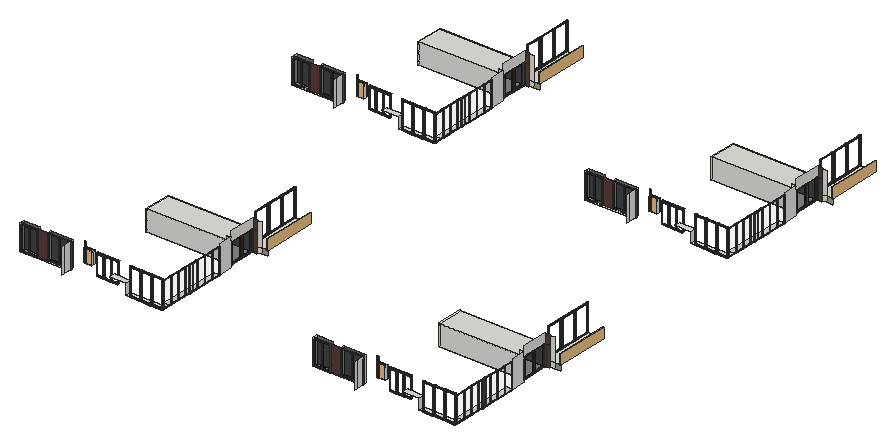
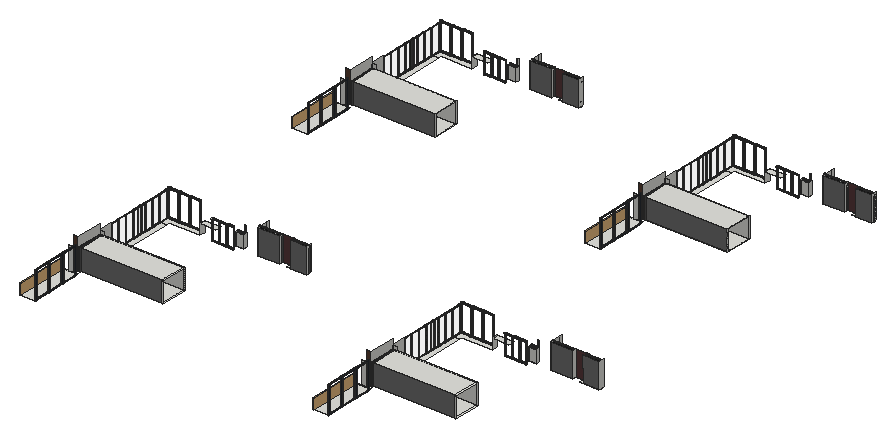
# SketchUp Ruby script. Lengths in inches.
U = 1.inch
M = Sketchup.active_model
def pt(a) = Geom::Point3d.new(a.map { |v| v * U })
def face(e, loops, mat)
  f = e.add_face(loops[0].map { |a| pt(a) })
  loops[1..].each { |l| e.add_face(l.map { |a| pt(a) }).erase! }
  f.material = f.back_material = mat if mat
  f
end
# faces: each face lists its corners as indices into pts; further lists are holes
def faces(e, pts, list, mat = nil) = list.each { |f| face(e, (f[0].is_a?(Array) ? f : [f]).map { |l| l.map { |i| pts[i] } }, mat) }
# xy, xz, yz: faces in a plane at the given z, y or x. An outline is a flat list of corners, or four numbers for a rectangle; further outlines are holes
def ring(l) = l.size == 4 ? [[l[0], l[1]], [l[2], l[1]], [l[2], l[3]], [l[0], l[3]]] : l.each_slice(2).to_a
def flat(e, list, mat, &to3) = list.each { |f| face(e, (f[0].is_a?(Array) ? f : [f]).map { |l| ring(l).map { |u, v| to3.(u, v) } }, mat) }
def xy(e, z, list, mat = nil) = flat(e, list, mat) { |x, y| [x, y, z] }
def xz(e, y, list, mat = nil) = flat(e, list, mat) { |x, z| [x, y, z] }
def yz(e, x, list, mat = nil) = flat(e, list, mat) { |y, z| [x, y, z] }
def lines(e, pts, list) = list.each { |a, b| e.add_line(pt(pts[a]), pt(pts[b])) }
# prism: a flat outline (further loops are holes) pulled along v
def prism(e, loops, v, mat = nil)
  f = face(e, loops, mat); d = Geom::Vector3d.new(v.map { |x| x * U })
  f.pushpull(f.normal.samedirection?(d) ? d.length : -d.length)
end
def box(e, o, s, mat = nil) = prism(e, [[o, [o[0] + s[0], o[1], o[2]], [o[0] + s[0], o[1] + s[1], o[2]], [o[0], o[1] + s[1], o[2]]]], [0, 0, s[2]], mat)
def at(x, y, z, deg = 0) = Geom::Transformation.translation(pt([x, y, z])) * Geom::Transformation.rotation(ORIGIN, Z_AXIS, deg.degrees)
def axes(o, x, y, z) = Geom::Transformation.new([*x, 0, *y, 0, *z, 0, *pt(o).to_a, 1])
def part(name) = M.definitions.add(name)
# library, detail: a bought-in or finely detailed component or shape, given as its bounding box
def library(name, o, s) = part(name).tap { |d| box(d.entities, o, s) }
def detail(e, o, s) = box(e.add_group.entities, o, s)
def put(e, d, t, mat = nil) = e.add_instance(d, t).tap { |i| i.material = mat if mat }
def group(e, t, mat = nil) = e.add_group.tap { |g| g.transformation = t; g.material = mat if mat }.entities
root = M.entities
M.materials.add("Glass_Tinted_Gray").color = [0, 0, 0]
M.materials["Glass_Tinted_Gray"].alpha = 0.125
M.materials.add("Glazing").color = [128, 128, 128]
M.materials["Glazing"].alpha = 0.05
M.materials.add("Powdercoating").color = [41, 44, 40]
M.materials.add("Wine2").color = [0, 0, 0]
M.materials["Wine2"].alpha = 0
M.materials.add("[0130_Gainsboro]").color = [39, 45, 50]
M.materials.add("[0135_DarkGray]").color = [81, 81, 81]
M.materials.add("[Color M05]").color = [114, 114, 114]
M.materials.add("[Color M06]").color = [86, 86, 86]
M.materials.add("[Concrete Tile]").color = [165, 155, 133]
M.materials.add("[Granite Brown]").color = [89, 59, 61]
M.materials.add("[Granite Brown]1").color = [89, 63, 50]
M.materials.add("[Mirror 02]").color = [229, 229, 229]
M.materials.add("[Terrazzo Light Blue]").color = [196, 214, 227]
c1 = part("Group\#15")
xy(c1.entities,0,[[0,-55.94,0.71,45.94]])
xy(c1.entities,0.2,[[0,-55.94,0.47,45.94],[0.47,45.94,0.71,46.42]])
xy(c1.entities,2.36,[[0.47,-55.94,0.71,46.42]])
xz(c1.entities,-55.94,[[0,0,0.71,0,0.71,2.36,0.47,2.36,0.47,0.2,0,0.2]])
xz(c1.entities,45.94,[[0,0,0.71,0.2]])
xz(c1.entities,46.42,[[0.47,0.2,0.71,2.36]])
yz(c1.entities,0,[[-55.94,0,45.94,0.2]])
yz(c1.entities,0.47,[[-55.94,0.2,46.42,2.36]])
yz(c1.entities,0.71,[[-55.94,0,45.94,0,45.94,0.2,46.42,0.2,46.42,2.36,-55.94,2.36]])
c2 = part("Group\#7")
xy(c2.entities,0,[[0,-59.09,0.71,45.94]])
xy(c2.entities,0.2,[[0,-59.09,0.47,45.94],[0.47,45.94,0.71,46.42]])
xy(c2.entities,2.36,[[0.47,-59.09,0.71,46.42]])
xz(c2.entities,-59.09,[[0,0,0.71,0,0.71,2.36,0.47,2.36,0.47,0.2,0,0.2]])
xz(c2.entities,45.94,[[0,0,0.71,0.2]])
xz(c2.entities,46.42,[[0.47,0.2,0.71,2.36]])
yz(c2.entities,0,[[-59.09,0,45.94,0.2]])
yz(c2.entities,0.47,[[-59.09,0.2,46.42,2.36]])
yz(c2.entities,0.71,[[-59.09,0,45.94,0,45.94,0.2,46.42,0.2,46.42,2.36,-59.09,2.36]])
c3 = part("Group\#16")
prism(c3.entities,[[[0.47,-56.18,0.2],[0,-56.18,0.2],[0,-56.18,0],[0.71,-56.18,0],[0.71,-56.18,2.36],[0.47,-56.18,2.36]]],[0,28.68,0])
c4 = part("Group\#10")
box(c4.entities,[-0.73,0,0],[27.99,0.55,102.05])
c5 = part("Group\#18")
xy(c5.entities,0,[[0.47,-56.18,0.47,-55.47,0,-55.47,0,-28.21,1.18,-28.21,1.18,-56.18]])
xy(c5.entities,0.2,[[0.71,-56.18,1.18,-28.21],[0,-55.47,0.47,-28.21],[0.47,-28.21,0.71,-27.74]])
xy(c5.entities,2.36,[[0.47,-56.18,0.71,-27.74]])
xz(c5.entities,-56.18,[[0.47,0,1.18,0,1.18,0.2,0.71,0.2,0.71,2.36,0.47,2.36]])
xz(c5.entities,-55.47,[[0,0,0.47,0.2]])
xz(c5.entities,-28.21,[[0,0,1.18,0.2]])
xz(c5.entities,-27.74,[[0.47,0.2,0.71,2.36]])
yz(c5.entities,0,[[-55.47,0,-28.21,0.2]])
yz(c5.entities,0.47,[[-56.18,0,-55.47,0.2],[-56.18,0.2,-27.74,2.36]])
yz(c5.entities,0.71,[[-56.18,0.2,-27.74,2.36]])
yz(c5.entities,1.18,[[-56.18,0,-28.21,0.2]])
c6 = part("Group\#34")
xy(c6.entities,0,[[-20.45,0,7.76,1.22]])
xy(c6.entities,0.06,[[-20.39,0.06,7.7,1.22]])
xy(c6.entities,0.47,[[-19.98,0,7.28,0.06]])
xy(c6.entities,101.89,[[-19.98,0,7.28,0.06]])
xy(c6.entities,102.3,[[-20.39,0.06,7.7,1.22]])
xy(c6.entities,102.36,[[-20.45,0,7.76,1.22]])
xz(c6.entities,0,[[[-20.45,0,7.76,102.36],[-19.98,0.47,7.28,101.89]]])
xz(c6.entities,0.06,[[[-20.39,0.06,7.7,102.3],[-19.98,0.47,7.28,101.89]]])
xz(c6.entities,1.22,[[[-20.45,0,7.76,102.36],[-20.39,0.06,7.7,102.3]]])
yz(c6.entities,-20.45,[[0,0,1.22,102.36]])
yz(c6.entities,-20.39,[[0.06,0.06,1.22,102.3]])
yz(c6.entities,-19.98,[[0,0.47,0.06,101.89]])
yz(c6.entities,7.28,[[0,0.47,0.06,101.89]])
yz(c6.entities,7.7,[[0.06,0.06,1.22,102.3]])
yz(c6.entities,7.76,[[0,0,1.22,102.36]])
c7 = part("Group\#6")
put(c7.entities,c1,axes([27.97,0,7.875],[1,0,0],[0,0,-1],[0,1,0]),"Powdercoating")
put(c7.entities,c2,axes([0.71,0,6.8],[-1,0,0],[0,0,-0.97687],[0,1,0]),"Powdercoating")
put(c7.entities,c3,axes([-27.5,0,-38.07],[0,0,-1],[-1,0,0],[0,1,0]),"Powdercoating")
put(c7.entities,c4,at(1.12,0.35,-38.39),"Glazing")
put(c7.entities,c5,axes([-27.5,0,63.35],[0,0,1],[-1,0,0],[0,1,0]),"Powdercoating")
put(c7.entities,c6,at(20.6875,1.0625,-38.54),"Powdercoating")
c8 = part("Sliding door assembly")
put(c8.entities,c7,at(-1.18,4.5,38.86))
g1 = group(c8.entities,at(84.74,4.5,38.86))
put(g1,c1,axes([-27.97,0,7.875],[-1,0,0],[0,0,-1],[0,1,0]),"Powdercoating")
put(g1,c2,axes([-0.71,0,6.8],[1,0,0],[0,0,-0.97687],[0,1,0]),"Powdercoating")
put(g1,c3,axes([27.5,0,-38.07],[0,0,-1],[1,0,0],[0,1,0]),"Powdercoating")
put(g1,c4,axes([-1.12,0.35,-38.39],[-1,0,0],[0,1,0],[0,0,1]),"Glazing")
put(g1,c5,axes([27.5,0,63.35],[0,0,1],[1,0,0],[0,1,0]),"Powdercoating")
put(g1,c6,axes([-20.6875,1.0625,-38.54],[-1,0,0],[0,1,0],[0,0,1]),"Powdercoating")
g2 = group(c8.entities,at(56.0625,4.5,38.86))
put(g2,c1,axes([-27.97,0,7.875],[-1,0,0],[0,0,-1],[0,1,0]),"Powdercoating")
put(g2,c3,axes([27.5,0,-38.07],[0,0,-1],[1,0,0],[0,1,0]),"Powdercoating")
put(g2,c4,axes([-1.12,0.35,-38.39],[-1,0,0],[0,1,0],[0,0,1]),"Glazing")
put(g2,c5,axes([27.5,0,63.35],[0,0,1],[1,0,0],[0,1,0]),"Powdercoating")
put(g2,c6,axes([-20.6875,1.0625,-38.54],[-1,0,0],[0,1,0],[0,0,1]),"Powdercoating")
g3 = group(g2,at(-0.71,0,6.8),"Powdercoating")
xy(g3,-45.34,[[0.47,0.2,0.71,2.36]])
xy(g3,-44.88,[[0,0,0.71,0.2]])
xy(g3,57.73,[[0,0,0.71,0,0.71,2.36,0.47,2.36,0.47,0.2,0,0.2]])
xz(g3,0,[[0,-44.88,0.71,57.73]])
xz(g3,0.2,[[0.47,-45.34,0.71,-44.88],[0,-44.88,0.47,57.73]])
xz(g3,2.36,[[0.47,-45.34,0.71,57.73]])
yz(g3,0,[[0,-44.88,0.2,57.73]])
yz(g3,0.47,[[0.2,-45.34,2.36,57.73]])
yz(g3,0.71,[[0.2,-45.34,2.36,-45.34,2.36,57.73,0,57.73,0,-44.88,0.2,-44.88]])
put(c8.entities,c7,axes([-33.94,4.5,38.86],[1.14218,0,0],[0,1,0],[0,0,1]))
c9 = part("sliding door")
put(c9.entities,c8,at(0,-4.5,-0.08))
c10 = part("Framed glazing panel")
xy(c10.entities,0,[[0,-0.98,43.07,0],[0,0,43.07,1.4]],"[0130_Gainsboro]")
xy(c10.entities,0.3,[[0.3,-1.43,42.77,-0.98]],"[0130_Gainsboro]")
xy(c10.entities,2.95,[[2.95,-1.43,40.12,-0.63],[2.95,-0.63,40.12,0],[2.95,0,40.12,0.64],[2.95,0.64,40.12,1.4]],"[0130_Gainsboro]")
xy(c10.entities,3.54,[[3.54,-0.63,39.53,0],[3.54,0,39.53,0.64]],"[0130_Gainsboro]")
xy(c10.entities,111.8125,[[3.54,-0.63,39.53,0],[3.54,0,39.53,0.64]],"[0130_Gainsboro]")
xy(c10.entities,112.4,[[2.95,-1.43,40.12,-0.63],[2.95,-0.63,40.12,0],[2.95,0,40.12,0.64],[2.95,0.64,40.12,1.4]],"[0130_Gainsboro]")
xy(c10.entities,115.05,[[0.3,-1.43,42.77,-0.98]],"[0130_Gainsboro]")
xy(c10.entities,115.35,[[0,-0.98,43.07,0],[0,0,43.07,1.4]],"[0130_Gainsboro]")
xz(c10.entities,-1.43,[[[0.3,0.3,42.77,115.05],[2.95,2.95,40.12,112.4]]],"[0130_Gainsboro]")
xz(c10.entities,-0.98,[[[0,0,43.07,115.35],[0.3,0.3,42.77,115.05]]],"[0130_Gainsboro]")
xz(c10.entities,-0.63,[[[2.95,2.95,40.12,112.4],[3.54,3.54,39.53,111.8125]]],"[0130_Gainsboro]")
xz(c10.entities,0,[[3.54,3.54,39.53,111.8125]],"Wine2")
xz(c10.entities,0,[[[0,0,43.07,115.35],[2.95,2.95,40.12,112.4]],[[2.95,2.95,40.12,112.4],[3.54,3.54,39.53,111.8125]]],"[0130_Gainsboro]")
xz(c10.entities,0.64,[[[2.95,2.95,40.12,112.4],[3.54,3.54,39.53,111.8125]]],"[0130_Gainsboro]")
xz(c10.entities,1.4,[[[0,0,43.07,115.35],[2.95,2.95,40.12,112.4]]],"[0130_Gainsboro]")
yz(c10.entities,0,[[-0.98,0,0,115.35],[0,0,1.4,115.35]],"[0130_Gainsboro]")
yz(c10.entities,0.3,[[-1.43,0.3,-0.98,115.05]],"[0130_Gainsboro]")
yz(c10.entities,2.95,[[-1.43,2.95,-0.63,112.4],[-0.63,2.95,0,112.4],[0,2.95,0.64,112.4],[0.64,2.95,1.4,112.4]],"[0130_Gainsboro]")
yz(c10.entities,3.54,[[-0.63,3.54,0,111.8125],[0,3.54,0.64,111.8125]],"[0130_Gainsboro]")
yz(c10.entities,39.53,[[-0.63,3.54,0,111.8125],[0,3.54,0.64,111.8125]],"[0130_Gainsboro]")
yz(c10.entities,40.12,[[-1.43,2.95,-0.63,112.4],[-0.63,2.95,0,112.4],[0,2.95,0.64,112.4],[0.64,2.95,1.4,112.4]],"[0130_Gainsboro]")
yz(c10.entities,42.77,[[-1.43,0.3,-0.98,115.05]],"[0130_Gainsboro]")
yz(c10.entities,43.07,[[-0.98,0,0,115.35],[0,0,1.4,115.35]],"[0130_Gainsboro]")
c11 = part("Glazed panel assembly")
put(c11.entities,c10,axes([90.57,1.43,0],[1.05148,0,0],[0,1,0],[0,0,1]))
put(c11.entities,c10,axes([0,1.43,0],[1.05148,0,0],[0,1,0],[0,0,1]))
put(c11.entities,c10,axes([45.29,1.43,0],[1.05148,0,0],[0,1,0],[0,0,1]))
c12 = part("PENTEK_RP Fineline 50S_Sliding_DoorCase_E1")
box(c12.entities,[0,0,0],[1.51,3.66,99.27],"[0135_DarkGray]")
c13 = part("PENTEK_RP Fineline 50S_SlidingDooe_Case_E2")
box(c13.entities,[0,0,0],[96.25,3.66,1.51],"[0135_DarkGray]")
c14 = part("pentek_RP Fineline 50S_SlidingDoor_Case")
put(c14.entities,c12,at(97.76,0,0))
put(c14.entities,c13,at(1.51,0,0))
put(c14.entities,c12,at(0,0,0))
put(c14.entities,c13,at(1.51,0,97.76))
c15 = part("PENTEK_RP Fineline 50S_SlidingDoor_GlazingBead_2")
box(c15.entities,[0,0,0],[0.56,0.59,94.39],"[0135_DarkGray]")
c16 = part("PENTEK_RP Fineline 50S_SlidingDoor_Glass")
box(c16.entities,[0,0,0],[46.58,0.16,94.39],"Glass_Tinted_Gray")
c17 = part("PENTEK_RP Fineline 50S_SlidingDoor_GlazingBead")
box(c17.entities,[0,0,0],[45.47,0.59,0.56],"[0135_DarkGray]")
c18 = part("PENTEK_RP Fineline 50S_SlidingDoor_Leaf_E1")
xy(c18.entities,0,[[0,0,0.93,1.97],[0.93,1.57,1.49,1.97]],"[0135_DarkGray]")
xy(c18.entities,96.25,[[0,0,0.93,0,0.93,1.57,1.49,1.57,1.49,1.97,0,1.97]],"[0135_DarkGray]")
xz(c18.entities,0,[[0,0,0.93,96.25]],"[0135_DarkGray]")
xz(c18.entities,1.57,[[0.93,0,1.49,95.32],[0.93,95.32,1.49,96.25]],"[0135_DarkGray]")
xz(c18.entities,1.97,[[0,0,1.49,96.25]],"[0135_DarkGray]")
yz(c18.entities,0,[[0,0,1.97,96.25]],"[0135_DarkGray]")
yz(c18.entities,0.93,[[0,0,1.57,0.93],[0,0.93,1.57,95.32],[0,95.32,1.57,96.25]],"[0135_DarkGray]")
yz(c18.entities,1.49,[[1.57,0,1.97,95.32],[1.57,95.32,1.97,96.25]],"[0135_DarkGray]")
c19 = part("PENTEK_RP Fineline 50S_SlidingDoor_Leaf_E2")
xy(c19.entities,0,[[0,0,0,1.57,0.56,1.57,0.56,1.97,46.02,1.97,46.02,1.57,46.58,1.57,46.58,0]],"[0135_DarkGray]")
xy(c19.entities,0.93,[[0,0,46.58,1.57]],"[0135_DarkGray]")
xy(c19.entities,1.49,[[0.56,1.57,46.02,1.97]],"[0135_DarkGray]")
xz(c19.entities,0,[[0,0,46.58,0.93]],"[0135_DarkGray]")
xz(c19.entities,1.57,[[0,0,0.56,0.93],[46.02,0,46.58,0.93],[0.56,0.93,46.02,1.49]],"[0135_DarkGray]")
xz(c19.entities,1.97,[[0.56,0,46.02,1.49]],"[0135_DarkGray]")
yz(c19.entities,0,[[0,0,1.57,0.93]],"[0135_DarkGray]")
yz(c19.entities,0.56,[[1.57,0,1.97,0.93],[1.57,0.93,1.97,1.49]],"[0135_DarkGray]")
yz(c19.entities,46.02,[[1.57,0,1.97,0.93],[1.57,0.93,1.97,1.49]],"[0135_DarkGray]")
yz(c19.entities,46.58,[[0,0,1.57,0.93]],"[0135_DarkGray]")
c20 = part("PENTEK_RP Fineline S_SlidingDoor_Leaf1")
put(c20.entities,c15,at(0.93,0,0.93))
put(c20.entities,c15,at(46.96,0,0.93))
put(c20.entities,c16,at(1.49,1.42,0.93))
put(c20.entities,c17,at(1.49,0,0.93))
put(c20.entities,c16,at(1.49,0.59,0.93),"[Terrazzo Light Blue]")
put(c20.entities,c18,at(0,0,0))
put(c20.entities,c18,axes([48.44,0,0],[-1,0,0],[0,1,0],[0,0,1]))
put(c20.entities,c19,axes([0.93,0,96.25],[1,0,0],[0,1,0],[0,0,-1]))
put(c20.entities,c19,at(0.93,0,0))
put(c20.entities,c17,at(1.49,0,94.77))
c21 = part("PENTEK_RP Fineline 50S_SlidingDoor_Leaf2")
put(c21.entities,c16,at(1.49,1.42,0.93))
put(c21.entities,c17,at(1.49,0,94.77))
put(c21.entities,c15,at(46.96,0,0.93))
put(c21.entities,c16,at(1.49,0.59,0.93),"[Mirror 02]")
put(c21.entities,c15,at(0.93,0,0.93))
put(c21.entities,c18,at(0,0,0))
put(c21.entities,c18,axes([48.44,0,0],[-1,0,0],[0,1,0],[0,0,1]))
put(c21.entities,c17,at(1.49,0,0.93))
put(c21.entities,c19,axes([0.93,0,96.25],[1,0,0],[0,1,0],[0,0,-1]))
put(c21.entities,c19,at(0.93,0,0))
c22 = part("PENTEK - Slimmest Steel Sliding Door / Window\#1")
put(c22.entities,c14,at(0,-1.88,-0.09))
put(c22.entities,c20,at(1.51,-2.27,1.42))
put(c22.entities,c21,at(49.32,-0.3,1.42))
c23 = library("Glass Railing",[0,0,0],[139.5,4.76,42])
c24 = library("Klein+raam",[128.36,12.7,0],[19.68,5.51,55.12])
xy(root,391.25,[[762.28,1799.9375,913.875,1799.9375,913.875,1835.1875,890.875,1835.1875,890.875,1822.9375,762.28,1822.9375],[1980.47,1799.9375,2132.0625,1799.9375,2132.0625,1835.1875,2109.0625,1835.1875,2109.0625,1822.9375,1980.47,1822.9375],[890.875,1835.1875,913.875,2095.79],[2109.0625,1835.1875,2132.0625,2095.79],[762.28,3214.625,913.875,3214.625,913.875,3249.875,890.875,3249.875,890.875,3237.625,762.28,3237.625],
  [1980.47,3214.625,2132.0625,3214.625,2132.0625,3249.875,2109.0625,3249.875,2109.0625,3237.625,1980.47,3237.625],[890.875,3249.875,913.875,3510.48],[2109.0625,3249.875,2132.0625,3510.48]])
xy(root,399.4375,[[319.53,1799.9375,523.04,1799.9375,523.04,1822.9375,431.33,1822.9375,431.33,1806.5625,400.54,1806.5625,400.54,1822.9375,319.53,1822.9375],[1537.72,1799.9375,1741.23,1799.9375,1741.23,1822.9375,1649.52,1822.9375,1649.52,1806.5625,1618.73,1806.5625,1618.73,1822.9375,1537.72,1822.9375],[319.53,3214.625,523.04,3214.625,523.04,3237.625,431.33,3237.625,431.33,3221.25,400.54,3221.25,400.54,3237.625,319.53,3237.625],[1537.72,3214.625,1741.23,3214.625,1741.23,3237.625,1649.52,3237.625,1649.52,3221.25,1618.73,3221.25,1618.73,3237.625,1537.72,3237.625]])
xy(root,401.36,[[560,2156.01,564.5,2266.33],[564.5,2156.01,913.875,2266.33],[1778.1875,2156.01,1782.6875,2266.33],[1782.6875,2156.01,2132.0625,2266.33],[560,3570.7,564.5,3681.01],
  [564.5,3570.7,913.875,3681.01],[1778.1875,3570.7,1782.6875,3681.01],[1782.6875,3570.7,2132.0625,3681.01]])
xy(root,408.0625,[[890.875,2295.875,954.6875,2518.89],[2109.0625,2295.875,2172.875,2518.89],[890.875,3710.5625,954.6875,3933.57],[2109.0625,3710.5625,2172.875,3933.57]])
xy(root,424.93,[[557.4,1837.8125,557.4,1850.5,589.71,1850.5,589.71,1847.4375,564.5,1847.4375,564.5,1837.8125],[564.5,1837.8125,589.71,1847.4375],[1775.59,1837.8125,1775.59,1850.5,1807.9,1850.5,1807.9,1847.4375,1782.6875,1847.4375,1782.6875,1837.8125],[1782.6875,1837.8125,1807.9,1847.4375],[557.4,3252.5,557.4,3265.1875,589.71,3265.1875,589.71,3262.125,564.5,3262.125,564.5,3252.5],
  [564.5,3252.5,589.71,3262.125],[1775.59,3252.5,1775.59,3265.1875,1807.9,3265.1875,1807.9,3262.125,1782.6875,3262.125,1782.6875,3252.5],[1782.6875,3252.5,1807.9,3262.125]])
xy(root,435.5,[[695.43,1799.9375,762.28,1822.9375],[1913.62,1799.9375,1980.47,1822.9375],[695.43,3214.625,762.28,3237.625],[1913.62,3214.625,1980.47,3237.625]])
xy(root,477.21,[[557.4,1837.8125,564.5,1837.8125,564.5,1847.4375,589.71,1847.4375,589.71,1850.5,557.4,1850.5],[564.5,1837.8125,589.71,1847.4375],[1775.59,1837.8125,1782.6875,1837.8125,1782.6875,1847.4375,1807.9,1847.4375,1807.9,1850.5,1775.59,1850.5],[1782.6875,1837.8125,1807.9,1847.4375],[557.4,3252.5,564.5,3252.5,564.5,3262.125,589.71,3262.125,589.71,3265.1875,557.4,3265.1875],
  [564.5,3252.5,589.71,3262.125],[1775.59,3252.5,1782.6875,3252.5,1782.6875,3262.125,1807.9,3262.125,1807.9,3265.1875,1775.59,3265.1875],[1782.6875,3252.5,1807.9,3262.125]])
xy(root,481.8125,[[611.65,1835.1875,701.59,1839.6875],[1829.84,1835.1875,1919.77,1839.6875],[611.65,3249.875,701.59,3254.375],[1829.84,3249.875,1919.77,3254.375]])
xy(root,487.04,[[560,2156.01,564.5,2266.33],[564.5,2156.01,913.875,2266.33],[1778.1875,2156.01,1782.6875,2266.33],[1782.6875,2156.01,2132.0625,2266.33],[560,3570.7,564.5,3681.01],
  [564.5,3570.7,913.875,3681.01],[1778.1875,3570.7,1782.6875,3681.01],[1782.6875,3570.7,2132.0625,3681.01]])
xz(root,1806.5625,[[400.54,399.4375,431.33,399.4375,431.33,504,401.14,504,386.33,504.07,385.81,399.51],[1618.73,399.4375,1649.52,399.4375,1649.52,504,1619.33,504,1604.52,504.07,1604,399.51]],"[Granite Brown]")
xz(root,1822.9375,[[319.53,399.4375,385.81,399.4375,386.33,504,319.53,504],[431.33,399.4375,523.04,504],[1537.72,399.4375,1604,399.4375,1604.52,504,1537.72,504],[1649.52,399.4375,1741.23,504]],"[Color M05]")
xz(root,1837.8125,[[557.88,424.93,560,477.21],[560,424.93,564.5,477.21],[1776.07,424.93,1778.1875,477.21],[1778.1875,424.93,1782.6875,477.21],[557.88,477.21,560,504],
  [560,477.21,564.5,504],[1776.07,477.21,1778.1875,504],[1778.1875,477.21,1782.6875,504]])
xz(root,1837.8125,[[557.4,424.93,557.88,477.21],[1775.59,424.93,1776.07,477.21]],"[Granite Brown]")
xz(root,1847.4375,[[564.5,424.93,589.71,477.21],[1782.6875,424.93,1807.9,477.21]])
xz(root,1850.5,[[557.4,424.93,589.71,477.21],[1775.59,424.93,1807.9,477.21]])
xz(root,2156.01,[[560,401.36,564.5,487.04],[564.5,401.36,894.3125,487.04],[894.3125,401.36,913.875,487.04],[1778.1875,401.36,1782.6875,487.04],[1782.6875,401.36,2112.5,487.04],
  [2112.5,401.36,2132.0625,487.04],[2112.5,401.36,2132.0625,487.04],[894.3125,487.04,913.875,504],[2112.5,487.04,2132.0625,504]])
xz(root,2266.33,[[560,401.36,564.5,487.04],[1778.1875,401.36,1782.6875,487.04]])
xz(root,2266.33,[[564.5,401.36,913.875,487.04],[1782.6875,401.36,2132.0625,487.04]],"[Color M05]")
xz(root,2266.33,[[913.875,401.36,930.75,487.04],[2132.0625,401.36,2148.9375,487.04],[913.875,487.04,930.75,527.36],[2132.0625,487.04,2148.9375,527.36]],"[Granite Brown]1")
xz(root,2295.875,[[913.875,385.75,930.75,408.0625],[2132.0625,385.75,2148.9375,408.0625],[913.875,408.0625,930.75,504],[2132.0625,408.0625,2148.9375,504]])
xz(root,2295.875,[[930.75,385.75,954.6875,408.0625],[2148.9375,385.75,2172.875,408.0625]],"[Concrete Tile]")
xz(root,3221.25,[[400.54,399.4375,431.33,399.4375,431.33,504,401.14,504,386.33,504.07,385.81,399.51],[1618.73,399.4375,1649.52,399.4375,1649.52,504,1619.33,504,1604.52,504.07,1604,399.51]],"[Granite Brown]")
xz(root,3237.625,[[319.53,399.4375,385.81,399.4375,386.33,504,319.53,504],[431.33,399.4375,523.04,504],[1537.72,399.4375,1604,399.4375,1604.52,504,1537.72,504],[1649.52,399.4375,1741.23,504]],"[Color M05]")
xz(root,3252.5,[[557.88,424.93,560,477.21],[560,424.93,564.5,477.21],[1776.07,424.93,1778.1875,477.21],[1778.1875,424.93,1782.6875,477.21],[557.88,477.21,560,504],
  [560,477.21,564.5,504],[1776.07,477.21,1778.1875,504],[1778.1875,477.21,1782.6875,504]])
xz(root,3252.5,[[557.4,424.93,557.88,477.21],[1775.59,424.93,1776.07,477.21]],"[Granite Brown]")
xz(root,3262.125,[[564.5,424.93,589.71,477.21],[1782.6875,424.93,1807.9,477.21]])
xz(root,3265.1875,[[557.4,424.93,589.71,477.21],[1775.59,424.93,1807.9,477.21]])
xz(root,3570.7,[[560,401.36,564.5,487.04],[564.5,401.36,894.3125,487.04],[894.3125,401.36,913.875,487.04],[1778.1875,401.36,1782.6875,487.04],[1782.6875,401.36,2112.5,487.04],
  [2112.5,401.36,2132.0625,487.04],[894.3125,487.04,913.875,504],[2112.5,487.04,2132.0625,504]])
xz(root,3681.01,[[560,401.36,564.5,487.04],[1778.1875,401.36,1782.6875,487.04]])
xz(root,3681.01,[[564.5,401.36,913.875,487.04],[1782.6875,401.36,2132.0625,487.04]],"[Color M05]")
xz(root,3681.01,[[913.875,401.36,930.75,487.04],[2132.0625,401.36,2148.9375,487.04],[913.875,487.04,930.75,527.36],[2132.0625,487.04,2148.9375,527.36]],"[Granite Brown]1")
xz(root,3710.5625,[[913.875,385.75,930.75,408.0625],[2132.0625,385.75,2148.9375,408.0625],[913.875,408.0625,930.75,504],[2132.0625,408.0625,2148.9375,504]])
xz(root,3710.5625,[[930.75,385.75,954.6875,408.0625],[2148.9375,385.75,2172.875,408.0625]],"[Concrete Tile]")
yz(root,319.53,[[1799.9375,399.4375,1822.9375,504],[3214.625,399.4375,3237.625,504]])
yz(root,431.33,[[1806.5625,399.4375,1822.9375,504],[3221.25,399.4375,3237.625,504]])
yz(root,523.04,[[1763.25,399.4375,1822.9375,504],[3177.9375,399.4375,3237.625,504]])
yz(root,557.4,[[1837.8125,424.93,1850.5,477.21],[3252.5,424.93,3265.1875,477.21]])
yz(root,564.5,[[1837.8125,424.93,1838.5625,477.21],[1838.5625,424.93,1847.4375,477.21],[3252.5,424.93,3253.25,477.21],[3253.25,424.93,3262.125,477.21],[1837.8125,477.21,1838.5625,504],
  [3252.5,477.21,3253.25,504]])
yz(root,589.71,[[1837.8125,424.93,1847.4375,477.21],[1847.4375,424.93,1850.5,477.21],[3252.5,424.93,3262.125,477.21],[3262.125,424.93,3265.1875,477.21]])
yz(root,762.28,[[1799.9375,391.25,1822.9375,435.5],[3214.625,391.25,3237.625,435.5]])
yz(root,913.875,[[2095.79,391.25,2156.01,504],[3510.48,391.25,3570.7,504],[2156.01,487.04,2266.33,527.36],[3570.7,487.04,3681.01,527.36]])
yz(root,1537.72,[[1799.9375,399.4375,1822.9375,504],[3214.625,399.4375,3237.625,504]])
yz(root,1649.52,[[1806.5625,399.4375,1822.9375,504],[3221.25,399.4375,3237.625,504]])
yz(root,1741.23,[[1763.25,399.4375,1822.9375,504],[3177.9375,399.4375,3237.625,504]])
yz(root,1775.59,[[1837.8125,424.93,1850.5,477.21],[3252.5,424.93,3265.1875,477.21]])
yz(root,1782.6875,[[1837.8125,424.93,1838.5625,477.21],[1838.5625,424.93,1847.4375,477.21],[3252.5,424.93,3253.25,477.21],[3253.25,424.93,3262.125,477.21],[1837.8125,477.21,1838.5625,504],
  [3252.5,477.21,3253.25,504]])
yz(root,1807.9,[[1837.8125,424.93,1847.4375,477.21],[1847.4375,424.93,1850.5,477.21],[3252.5,424.93,3262.125,477.21],[3262.125,424.93,3265.1875,477.21]])
yz(root,1980.47,[[1799.9375,391.25,1822.9375,435.5],[3214.625,391.25,3237.625,435.5]])
yz(root,2132.0625,[[2095.79,391.25,2156.01,504],[3510.48,391.25,3570.7,504],[2156.01,487.04,2266.33,527.36],[3570.7,487.04,3681.01,527.36]])
p = [[1741.23,1778.3125,399.4375],[1741.23,1778.3125,504],[2132.0625,2156.01,391.25],[2132.0625,2156.65,391.25],[523.04,1778.3125,399.4375],[523.04,1778.3125,504],
  [913.875,2156.01,391.25],[913.875,2156.65,391.25],[1741.23,3193,399.4375],[1741.23,3193,504],[2132.0625,3570.7,391.25],[2132.0625,3571.34,391.25],
  [913.875,3570.7,391.25],[913.875,3571.34,391.25],[523.04,3193,399.4375],[523.04,3193,504]]
lines(root,p,[[0,1],[2,3],[4,5],[6,7],[8,9],[10,11],[12,13],[14,15]])
put(root,c9,axes([2135.49,1979.63,391],[0,1.302,0],[-1,0,0],[0,0,1.03877]))
put(root,c9,axes([917.3,1979.63,391],[0,1.302,0],[-1,0,0],[0,0,1.03877]))
put(root,c9,axes([2135.49,3394.32,391],[0,1.302,0],[-1,0,0],[0,0,1.03877]))
put(root,c9,axes([917.3,3394.32,391],[0,1.302,0],[-1,0,0],[0,0,1.03877]))
put(root,c9,axes([2134.42,1844.13,391.25],[0,1.302,0],[-1,0,0],[0,0,1.03877]))
put(root,c9,axes([916.24,1844.13,391.25],[0,1.302,0],[-1,0,0],[0,0,1.03877]))
put(root,c9,axes([2134.42,3258.81,391.25],[0,1.302,0],[-1,0,0],[0,0,1.03877]))
put(root,c9,axes([916.24,3258.81,391.25],[0,1.302,0],[-1,0,0],[0,0,1.03877]))
put(root,c11,at(1996.2,1797.11,391.25))
put(root,c11,at(778.01,1797.11,391.25))
put(root,c11,at(1996.2,3211.79,391.25))
put(root,c11,at(778.01,3211.79,391.25))
put(root,c11,axes([1829.4375,1833.46,395.3125],[0.6649,0,0],[0,0.61,0],[0,0,0.74986]),"[Color M06]")
put(root,c11,axes([611.25,1833.46,395.3125],[0.6649,0,0],[0,0.61,0],[0,0,0.74986]),"[Color M06]")
put(root,c11,axes([1829.4375,3248.15,395.3125],[0.6649,0,0],[0,0.61,0],[0,0,0.74986]),"[Color M06]")
put(root,c11,axes([611.25,3248.15,395.3125],[0.6649,0,0],[0,0.61,0],[0,0,0.74986]),"[Color M06]")
put(root,c22,axes([1537.72,1806.83,397.03],[0.69114,0,0],[0,0.88,0],[0,0,1.054]))
put(root,c22,axes([319.53,1806.83,397.03],[0.69114,0,0],[0,0.88,0],[0,0,1.054]))
put(root,c22,axes([1537.72,3221.52,397.03],[0.69114,0,0],[0,0.88,0],[0,0,1.054]))
put(root,c22,axes([319.53,3221.52,397.03],[0.69114,0,0],[0,0.88,0],[0,0,1.054]))
put(root,c22,axes([1649.52,1808.21,399.53],[0.95582,0,0],[0,0.88,0],[0,0,1.054]))
put(root,c22,axes([431.33,1808.21,399.53],[0.95582,0,0],[0,0.88,0],[0,0,1.054]))
put(root,c22,axes([1649.52,3222.9,399.53],[0.95582,0,0],[0,0.88,0],[0,0,1.054]))
put(root,c22,axes([431.33,3222.9,399.53],[0.95582,0,0],[0,0.88,0],[0,0,1.054]))
put(root,c22,axes([2127.34,2156.65,400.11],[0,1.12181,0],[-2.51374,0,0],[0,0,0.87918]))
put(root,c22,axes([909.16,2156.65,400.11],[0,1.12181,0],[-2.51374,0,0],[0,0,0.87918]))
put(root,c22,axes([2127.34,3571.34,400.11],[0,1.12181,0],[-2.51374,0,0],[0,0,0.87918]))
put(root,c22,axes([909.16,3571.34,400.11],[0,1.12181,0],[-2.51374,0,0],[0,0,0.87918]))
put(root,c11,axes([2109.0625,2309.55,408.0625],[0,1.54079,0],[-1,0,0],[0,0,1]))
put(root,c23,axes([2172.875,2295.6875,408.0625],[0,1.6,0],[-1,0,0],[0,0,1]))
put(root,c23,axes([954.6875,2295.6875,408.0625],[0,1.6,0],[-1,0,0],[0,0,1]))
put(root,c11,axes([890.875,2309.55,408.0625],[0,1.54079,0],[-1,0,0],[0,0,1]))
put(root,c23,axes([2172.875,3710.375,408.0625],[0,1.6,0],[-1,0,0],[0,0,1]))
put(root,c11,axes([2109.0625,3724.24,408.0625],[0,1.54079,0],[-1,0,0],[0,0,1]))
put(root,c11,axes([890.875,3724.24,408.0625],[0,1.54079,0],[-1,0,0],[0,0,1]))
put(root,c23,axes([954.6875,3710.375,408.0625],[0,1.6,0],[-1,0,0],[0,0,1]))
put(root,c24,axes([1572.84,1829.18,424.93],[1.58777,0,0],[0,0.68,0],[0,0,0.99202]))
put(root,c24,axes([354.65,1829.18,424.93],[1.58777,0,0],[0,0.68,0],[0,0,0.99202]))
put(root,c24,axes([1572.84,3243.87,424.93],[1.58777,0,0],[0,0.68,0],[0,0,0.99202]))
put(root,c24,axes([354.65,3243.87,424.93],[1.58777,0,0],[0,0.68,0],[0,0,0.99202]))
